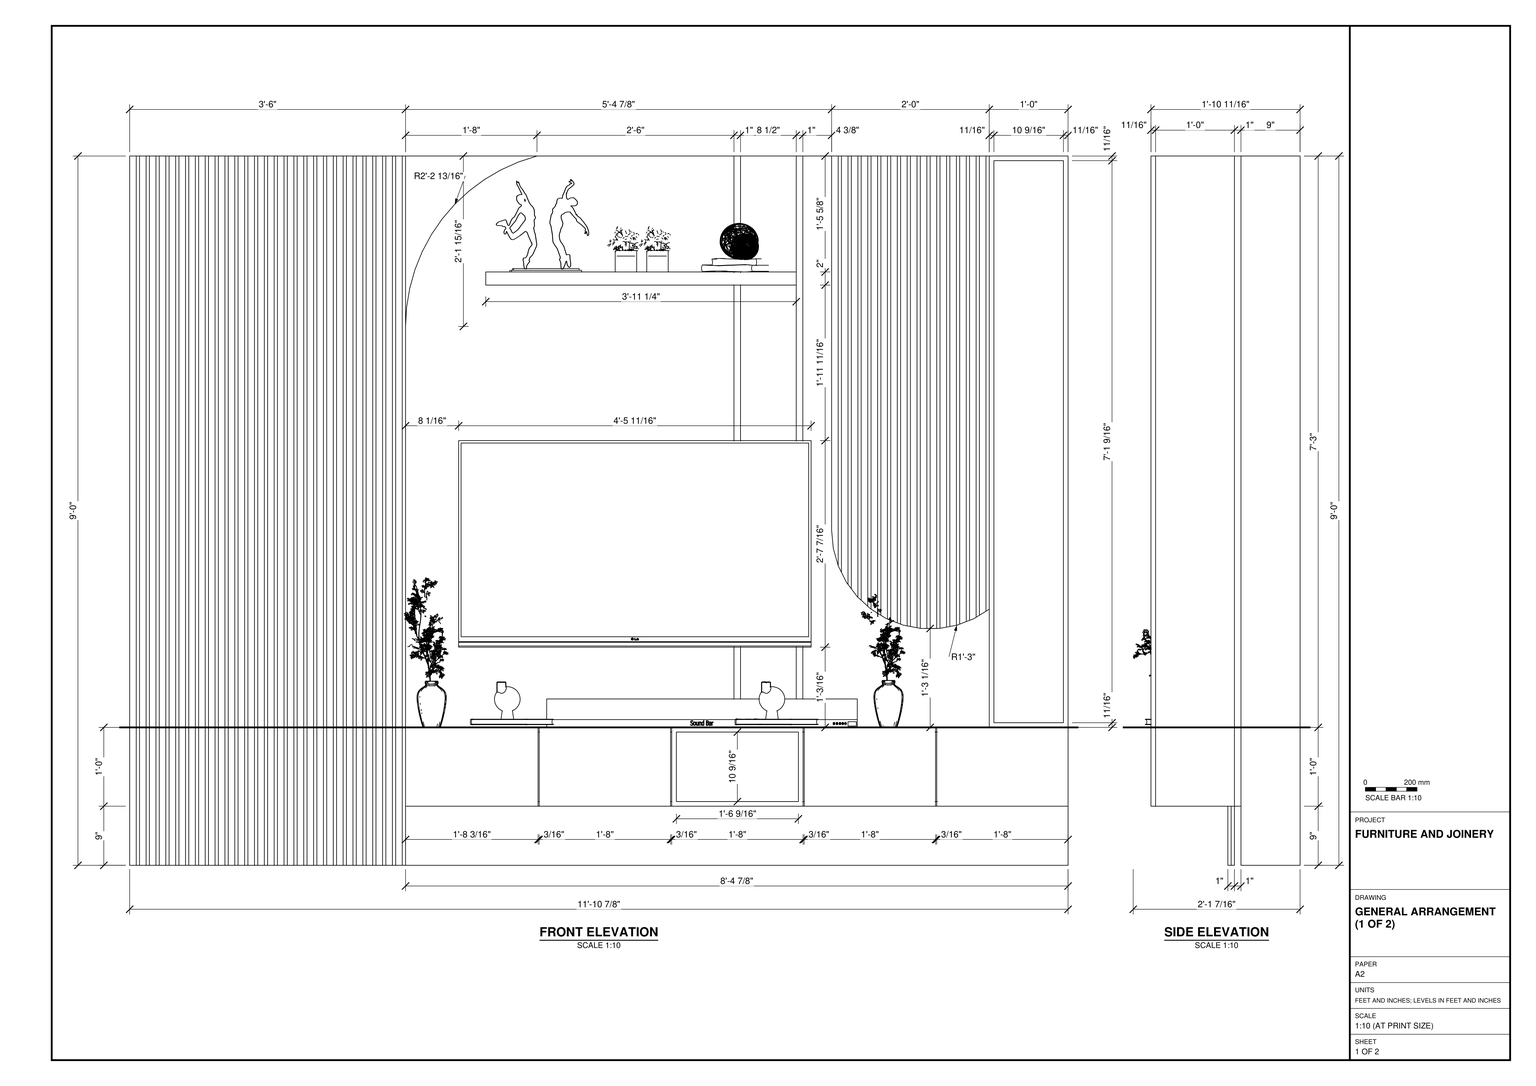
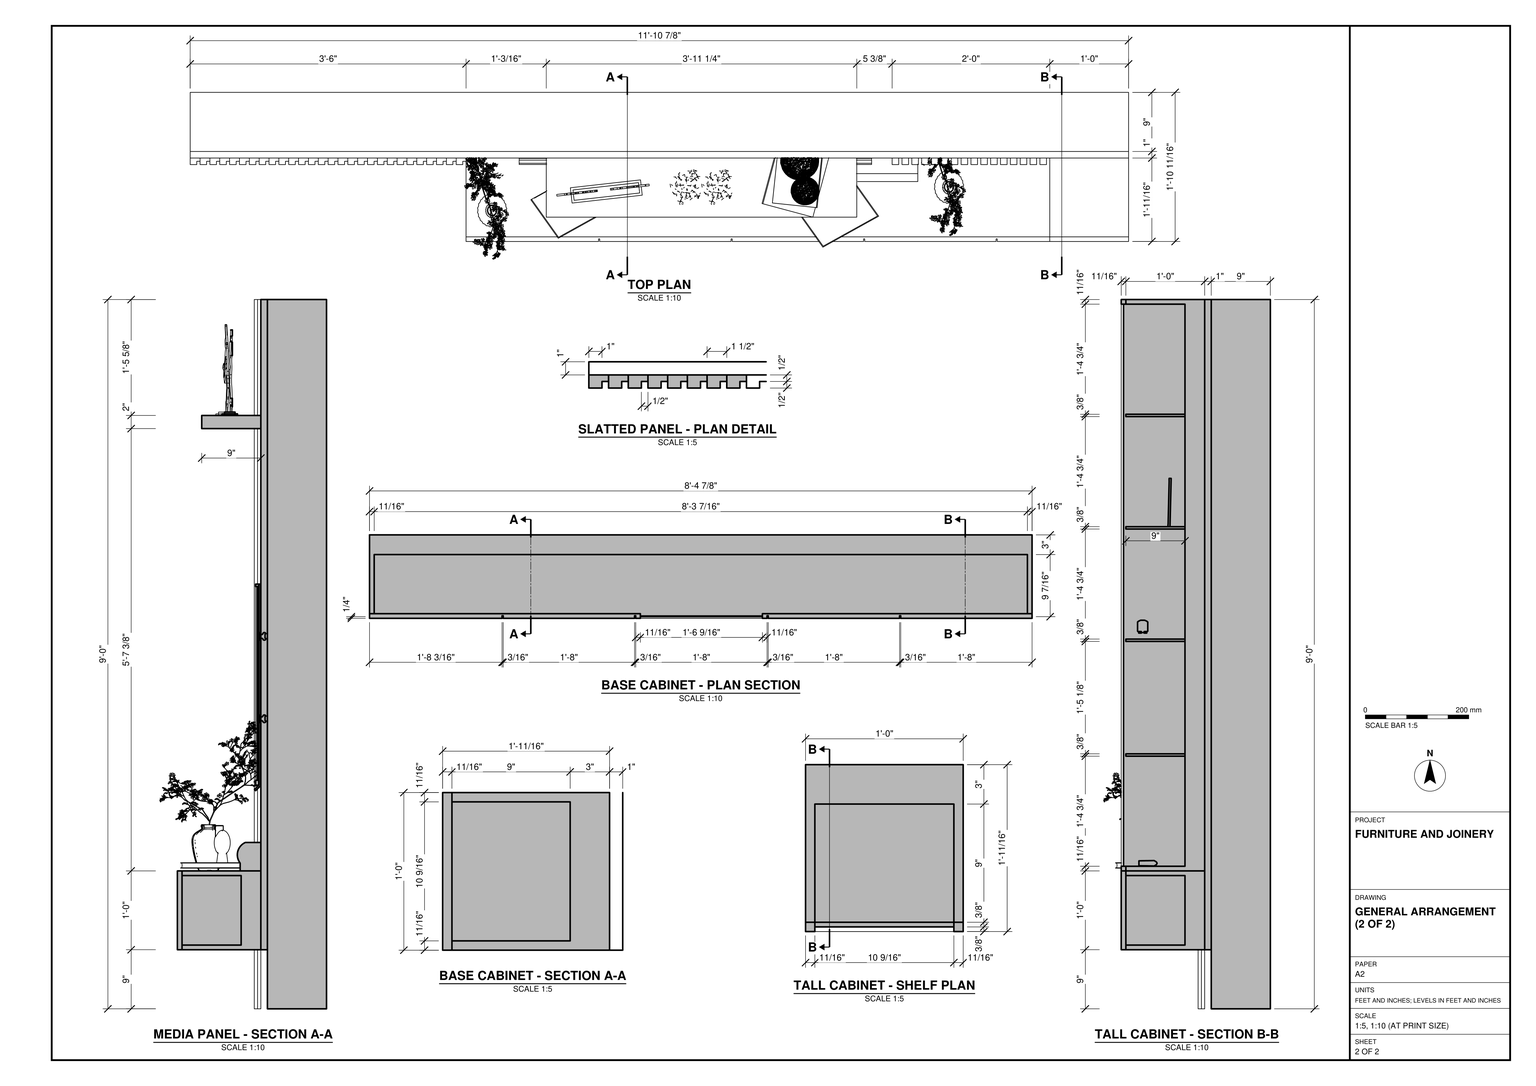
Build the media wall in SketchUp from task_files/diagram_01.pdf. Work in feet and inches, using the floor as the ±0'-0" datum. The complete assembly is 11'-10 7/8" wide, 2'-1 7/16" deep and 9'-0" high. Use the front elevation to set out the panels and cabinet faces, and the plan and sections to establish their depths.

Model the 9" thick backing wall and the full-height slatted panel at the left. Form the projecting slats and intervening grooves as shown in the plan detail. Reproduce the curved line at the upper left of the central media panel, its narrow vertical divisions and the curved lower edge of the slatted panel on the right. Fit the tall, narrow cabinet against the right end, with its framed front and internal shelves.

Run the suspended base cabinet from the left slatted panel to the right end. Include the gaps between its fronts and the inset centre bay. Position the television between the upper display shelf and the base cabinet, with the soundbar below the television. Decor and loose items on the shelf and cabinet may be any suitable library components. Keep the backing wall and each joinery or equipment piece in separate groups or components, and use components for repeated parts. Save one SketchUp model as output_files/media_wall_with_slatted_panels_and_fitted_cabinetry.skp.

# SketchUp Ruby script. Lengths in inches.
U = 1.inch
M = Sketchup.active_model
def pt(a) = Geom::Point3d.new(a.map { |v| v * U })
def face(e, loops, mat)
  f = e.add_face(loops[0].map { |a| pt(a) })
  loops[1..].each { |l| e.add_face(l.map { |a| pt(a) }).erase! }
  f.material = f.back_material = mat if mat
  f
end
# faces: each face lists its corners as indices into pts; further lists are holes
def faces(e, pts, list, mat = nil) = list.each { |f| face(e, (f[0].is_a?(Array) ? f : [f]).map { |l| l.map { |i| pts[i] } }, mat) }
# xy, xz, yz: faces in a plane at the given z, y or x. An outline is a flat list of corners, or four numbers for a rectangle; further outlines are holes
def ring(l) = l.size == 4 ? [[l[0], l[1]], [l[2], l[1]], [l[2], l[3]], [l[0], l[3]]] : l.each_slice(2).to_a
def flat(e, list, mat, &to3) = list.each { |f| face(e, (f[0].is_a?(Array) ? f : [f]).map { |l| ring(l).map { |u, v| to3.(u, v) } }, mat) }
def xy(e, z, list, mat = nil) = flat(e, list, mat) { |x, y| [x, y, z] }
def xz(e, y, list, mat = nil) = flat(e, list, mat) { |x, z| [x, y, z] }
def yz(e, x, list, mat = nil) = flat(e, list, mat) { |y, z| [x, y, z] }
def lines(e, pts, list) = list.each { |a, b| e.add_line(pt(pts[a]), pt(pts[b])) }
# prism: a flat outline (further loops are holes) pulled along v
def prism(e, loops, v, mat = nil)
  f = face(e, loops, mat); d = Geom::Vector3d.new(v.map { |x| x * U })
  f.pushpull(f.normal.samedirection?(d) ? d.length : -d.length)
end
def box(e, o, s, mat = nil) = prism(e, [[o, [o[0] + s[0], o[1], o[2]], [o[0] + s[0], o[1] + s[1], o[2]], [o[0], o[1] + s[1], o[2]]]], [0, 0, s[2]], mat)
def at(x, y, z, deg = 0) = Geom::Transformation.translation(pt([x, y, z])) * Geom::Transformation.rotation(ORIGIN, Z_AXIS, deg.degrees)
def axes(o, x, y, z) = Geom::Transformation.new([*x, 0, *y, 0, *z, 0, *pt(o).to_a, 1])
def part(name) = M.definitions.add(name)
# library, detail: a bought-in or finely detailed component or shape, given as its bounding box
def library(name, o, s) = part(name).tap { |d| box(d.entities, o, s) }
def detail(e, o, s) = box(e.add_group.entities, o, s)
def put(e, d, t, mat = nil) = e.add_instance(d, t).tap { |i| i.material = mat if mat }
def group(e, t, mat = nil) = e.add_group.tap { |g| g.transformation = t; g.material = mat if mat }.entities
root = M.entities
M.materials.add("C04_Amber_Sunshine").color = [255, 152, 49]
M.materials.add("Color_009").color = [0, 0, 0]
M.materials.add("Glass_Basic_01").color = [161, 173, 186]
M.materials["Glass_Basic_01"].alpha = 0.25
M.materials.add("M08_Obsidian_Black").color = [30, 30, 30]
M.materials.add("Plywood_01_1K").color = [125, 96, 64]
M.materials.add("[Color_000]2").color = [135, 140, 128]
c1 = library("Flat screen television",[0,8.92,0],[57.09,3.02,33.46])
c2 = library("Component114",[-82.06,-82.06,-129.5625],[164.12,164.12,259.1])
c3 = library("Component117",[-887.5,-1285.52,872.49],[3843.85,2719.29,5329.54])
c4 = library("Component119",[-554.81,-1390.41,779.52],[3610.96,2909.33,5473.88])
c5 = part("Component118")
put(c5.entities,c3,axes([-495.49,21.52,-677.71],[-0.13024,0.05973,0.15696],[-0.0368,-0.22453,0.01695],[0.17844,-0.01756,0.15474]))
put(c5.entities,c4,axes([-495.49,21.52,-677.71],[-0.13024,0.05973,0.15696],[-0.0368,-0.22453,0.01695],[0.17844,-0.01756,0.15474]))
c6 = part("Component116")
put(c6.entities,c2,axes([-124.16,15.74,-281.79],[-1.44088,0.62571,0],[-0.62571,-1.44088,0],[0,0,1.57088]))
put(c6.entities,c5,axes([19.67,96.68,265.57],[0.78615,0.27839,0],[0.27839,-0.78615,0],[0,0,0.83398]))
c7 = part("Component115")
put(c7.entities,c6,at(176.39,-15.27,-335.67))
c8 = library("Component124",[-34.71,-73.39,-113.66],[69.42,146.78,227.32])
c9 = library("Component126",[-109.42,-139.7,-27.27],[219.95,281.4,27.83])
c10 = library("Component128",[-218.98,-37.49,7.99],[213.01,261.68,22.71])
c11 = part("Component127")
put(c11.entities,c9,at(-0.56,-1,27.27))
put(c11.entities,c10,axes([112.41,-97.69,-5.43],[1,0,0],[0,1.0465,0],[0,0,1]))
c12 = part("Component125")
put(c12.entities,c8,axes([-16.9,-33.42,-7.27],[-0.38375,-0.70679,0],[-0.70679,0.38375,0],[0,0,0.80425]))
put(c12.entities,c11,axes([0,0,-117.43],[0.41792,0.87796,0],[0.87796,-0.41792,0],[0,0,0.97235]))
c13 = library("SoundBar",[0,0,0],[61.42,3.58,4.33])
c14 = library("dançarinos",[1.14,-1.57,0.12],[22.8,3.55,21.3])
c15 = library("Books and ornaments",[0,0,0],[11.85,7.68,6.68])
c16 = part("Group10\#1")
xy(c16.entities,0,[[-11,-26.41,-11.75,-23.78,-12,-21.03,-12,35.97,-11,35.97]])
xy(c16.entities,1,[[-11,-26.41,-11,35.97,-12,35.97,-12,-21.03,-11.75,-23.78]])
xz(c16.entities,35.97,[[-12,0,-11,1]])
yz(c16.entities,-12,[[-21.03,0,35.97,1]])
yz(c16.entities,-11,[[-26.41,0,35.97,1]])
c17 = part("Group11\#1")
xy(c17.entities,0,[[-9.5,-29.26,-9.76,-28.92,-10.5,-27.43,-10.5,35.97,-9.5,35.97]])
xy(c17.entities,1,[[-9.5,-29.26,-9.5,35.97,-10.5,35.97,-10.5,-27.43,-9.76,-28.92]])
xz(c17.entities,35.97,[[-10.5,0,-9.5,1]])
yz(c17.entities,-10.5,[[-27.43,0,35.97,1]])
yz(c17.entities,-9.5,[[-29.26,0,35.97,1]])
c18 = part("Group12\#1")
xy(c18.entities,0,[[-8,-31.21,-8.1,-31.125,-9,-29.92,-9,35.97,-8,35.97]])
xy(c18.entities,1,[[-8,-31.21,-8,35.97,-9,35.97,-9,-29.92,-8.1,-31.125]])
xz(c18.entities,35.97,[[-9,0,-8,1]])
yz(c18.entities,-9,[[-29.92,0,35.97,1]])
yz(c18.entities,-8,[[-31.21,0,35.97,1]])
c19 = part("Group13\#1")
prism(c19.entities,[[[-7.5,-31.67,0],[-7.5,35.97,0],[-6.5,35.97,0],[-6.5,-32.58,0]]],[0,0,1])
c20 = part("Group14\#1")
prism(c20.entities,[[[-6,-33.02,0],[-6,35.97,0],[-5,35.97,0],[-5,-33.64,0]]],[0,0,1])
c21 = part("Group15\#1")
xy(c21.entities,0,[[-3.5,-34.53,-3.71,-34.45,-4.5,-33.95,-4.5,35.97,-3.5,35.97]])
xy(c21.entities,1,[[-3.5,-34.53,-3.5,35.97,-4.5,35.97,-4.5,-33.95,-3.71,-34.45]])
xz(c21.entities,35.97,[[-4.5,0,-3.5,1]])
yz(c21.entities,-4.5,[[-33.95,0,35.97,1]])
yz(c21.entities,-3.5,[[-34.53,0,35.97,1]])
c22 = part("Group16\#1")
prism(c22.entities,[[[-3,-34.72,0],[-3,35.97,0],[-2,35.97,0],[-2,-35.11,0]]],[0,0,1])
c23 = part("Group17\#1")
xy(c23.entities,0,[[-0.5,-35.57,-1.13,-35.45,-1.5,-35.31,-1.5,35.97,-0.5,35.97]])
xy(c23.entities,1,[[-0.5,-35.57,-0.5,35.97,-1.5,35.97,-1.5,-35.31,-1.13,-35.45]])
yz(c23.entities,-1.5,[[-35.31,0,35.97,1]])
yz(c23.entities,-0.5,[[-35.57,0,35.97,1]])
c24 = part("Group18\#1")
prism(c24.entities,[[[1,35.97,0],[1,-35.85,0],[0,-35.66,0],[0,35.97,0]]],[0,0,1])
c25 = part("Group19\#1")
xy(c25.entities,0,[[2.5,-35.97,1.58,-35.96,1.5,-35.95,1.5,35.97,2.5,35.97]])
xy(c25.entities,1,[[2.5,-35.97,2.5,35.97,1.5,35.97,1.5,-35.95,1.58,-35.96]])
xz(c25.entities,35.97,[[1.5,0,2.5,1]])
yz(c25.entities,1.5,[[-35.95,0,35.97,1]])
yz(c25.entities,2.5,[[-35.97,0,35.97,1]])
c26 = part("Group20\#1")
box(c26.entities,[3,-35.97,0],[1,71.94,1])
c27 = part("Group21\#1")
prism(c27.entities,[[[4.5,-35.94,0],[4.5,35.97,0],[5.5,35.97,0],[5.5,-35.76,0]]],[0,0,1])
c28 = part("Group22\#1")
prism(c28.entities,[[[7,35.97,0],[7,-35.48,0],[6,-35.67,0],[6,35.97,0]]],[0,0,1])
c29 = part("Group23\#1")
prism(c29.entities,[[[8.5,35.97,0],[8.5,-34.92,0],[7.5,-35.3,0],[7.5,35.97,0]]],[0,0,1])
c30 = part("Group24\#1")
xy(c30.entities,0,[[9,-34.73,9,35.97,10,35.97,10,-34.26,9.65,-34.48]])
xy(c30.entities,1,[[9,-34.73,9.65,-34.48,10,-34.26,10,35.97,9,35.97]])
yz(c30.entities,9,[[-34.73,0,35.97,1]])
yz(c30.entities,10,[[-34.26,0,35.97,1]])
c31 = part("Group25\#1")
prism(c31.entities,[[[11.5,35.97,0],[11.5,-33.34,0],[10.5,-33.95,0],[10.5,35.97,0]]],[0,0,1])
c32 = part("Group26\#1")
yz(c32.entities,12,[[-33.03,0,35.97,1]])
c33 = part("Group8\#1")
put(c33.entities,c16,at(0,0,0))
put(c33.entities,c17,at(0,0,0))
put(c33.entities,c18,at(0,0,0))
put(c33.entities,c19,at(0,0,0))
put(c33.entities,c20,at(0,0,0))
put(c33.entities,c21,at(0,0,0))
put(c33.entities,c22,at(0,0,0))
put(c33.entities,c23,at(0,0,0))
put(c33.entities,c24,at(0,0,0))
put(c33.entities,c25,at(0,0,0))
put(c33.entities,c26,at(0,0,0))
put(c33.entities,c27,at(0,0,0))
put(c33.entities,c28,at(0,0,0))
put(c33.entities,c29,at(0,0,0))
put(c33.entities,c30,at(0,0,0))
put(c33.entities,c31,at(0,0,0))
put(c33.entities,c32,at(0,0,0))
c34 = part("Vertical wall slat")
xy(c34.entities,0,[[0,0,1,1],[1,0.5,1.5,1]])
xy(c34.entities,108,[[0,0,1,0,1,0.5,1.5,0.5,1.5,1,0,1]])
xz(c34.entities,0,[[0,0,1,108]])
xz(c34.entities,0.5,[[1,0,1.5,108]])
yz(c34.entities,0,[[0,0,1,108]])
yz(c34.entities,1,[[0,0,0.5,108]])
yz(c34.entities,1.5,[[0.5,0,1,108]])
c35 = part("Group\#9")
box(c35.entities,[0,0,0],[10.58,9,0.35])
c36 = library("Group7\#2",[0.82,-1.15,-0.02],[1.93,1.97,2.94])
c37 = library("Groupe\#10",[0,0,0],[43.68,4.59,18.71])
c38 = part("Agrupar\#3")
xy(c38.entities,21.7,[[0.99,0.93,21.68,0.97]])
yz(c38.entities,0,[[0.55,0,0,22.67,0.94,22.69,1.5,0.02]],"[Color_000]2")
yz(c38.entities,0.99,[[1.44,1.01,1.47,1.02,0.97,21.7,0.93,21.7]])
yz(c38.entities,21.68,[[1.44,1.01,0.93,21.7,0.97,21.7,1.47,1.02]])
yz(c38.entities,22.68,[[0.55,0,1.5,0.02,0.94,22.69,0,22.67]],"[Color_000]2")
p = [[0,0.55,0],[22.68,0.55,0],[22.68,0,22.67],[0,0,22.67],[0,1.5,0.02],[22.68,1.5,0.02],
  [0,0.94,22.69],[22.68,0.94,22.69],[21.68,1.47,1.02],[21.68,0.97,21.7],[0.99,0.97,21.7],[0.99,1.47,1.02],
  [21.68,0.93,21.7],[21.68,1.44,1.01],[0.99,1.44,1.01],[0.99,0.93,21.7]]
faces(c38.entities,p,[[0,1,2,3],[4,5,1,0],[7,6,3,2]],"[Color_000]2")
faces(c38.entities,p,[[[5,4,6,7],[8,9,10,11]],[12,13,14,15],[8,11,14,13]])
c39 = part("Agrupar\#30")
xy(c39.entities,14.62,[[0.51,0.6,16.18,0.64]])
yz(c39.entities,0,[[0.42,0,0,15.11,0.63,15.13,1.05,0.02]],"Color_009")
yz(c39.entities,0.51,[[1,0.52,1.04,0.53,0.64,14.62,0.6,14.62]])
yz(c39.entities,16.18,[[1,0.52,0.6,14.62,0.64,14.62,1.04,0.53]])
yz(c39.entities,16.69,[[0.42,0,1.05,0.02,0.63,15.13,0,15.11]],"Color_009")
p = [[0,0.42,0],[16.69,0.42,0],[16.69,0,15.11],[0,0,15.11],[16.69,1.05,0.02],[0,1.05,0.02],
  [0,0.63,15.13],[16.69,0.63,15.13],[16.18,0.64,14.62],[0.51,0.64,14.62],[0.51,1.04,0.53],[16.18,1.04,0.53],
  [0.51,0.6,14.62],[16.18,0.6,14.62],[16.18,1,0.52],[0.51,1,0.52]]
faces(c39.entities,p,[[0,1,2,3],[4,1,0,5],[2,7,6,3]],"Color_009")
faces(c39.entities,p,[[[4,5,6,7],[8,9,10,11]],[12,13,14,15],[11,10,15,14]])
c40 = library("Group\#263",[-0.77,-0.82,0],[7.28,10.35,17.46])
c41 = library("Group\#264",[0,0,0],[5.61,9.8,6.92])
put(root,c1,axes([103.75,22.95,33.21],[-0.94,0,0],[0,-0.94,0],[0,0,0.94]))
put(root,c7,axes([45.98,3.7,35.3],[0,0.01977,0],[-0.01747,0,0],[0,0,0.01747]))
put(root,c12,axes([58.2,5.79,25.2],[-0.01967,-0.02738,0],[0.03099,-0.01737,0],[0,0,0.03242]))
put(root,c7,axes([115.54,7.28,35.41],[0,0.01977,0],[-0.01747,0,0],[0,0,0.01747]))
put(root,c12,axes([98.49,4.43,25.2],[-0.01967,-0.02738,0],[0.03099,-0.01737,0],[0,0,0.03242]))
put(root,c13,axes([63.49,9.125,21],[0.77,0,0],[0,1,0],[0,0,1]))
put(root,c14,axes([70.6,8.5625,90.27],[-0.61653,-0.06916,0],[0.07357,-0.65589,0],[0,0,0.66]))
put(root,c15,axes([90.22,18.56,90.35],[-0.28729,-1.07218,0],[1.07218,-0.28729,0],[0,0,1.11]))
put(root,c15,axes([134.57,13.23,21.71],[-0.2327,-0.86846,0],[0.86846,-0.2327,0],[0,0,0.8991]))
g1 = group(root,at(0,13.71,0))
box(g1,[0,0,0],[142.87,9,108])
g2 = group(root,at(0,12.71,0))
xy(g2,9,[[0,0,142.87,1]])
xy(g2,108,[[0,0,142.87,1]])
xz(g2,0,[[0,9,42,108],[42,9,142.87,9,142.87,108,130.87,108,130.87,39,128.52,37.55,125.9375,36.5625,123.22,36.0625,120.45,36.07,117.74,36.58,115.16,37.58,112.82,39.04,110.78,40.91,109.11,43.11,107.88,45.59,107.125,48.25,106.87,51,106.87,108,102.49,108,102.49,21,101.49,21,101.49,108,93,108,93,21,92,21,92,108,62.01,108,59.22,107.1,56.54,105.9,54.01,104.41,51.65,102.66,49.5,100.66,47.59,98.4375,45.92,96.02,44.53,93.43,43.43,90.71,42.64,87.88,42.16,84.98,42,82.05],[123.22,36.0625,125.9375,36.5625,128.52,37.55,130.87,39,130.87,108,106.87,108,106.87,51,107.125,48.25,107.88,45.59,109.11,43.11,110.78,40.91,112.82,39.04,115.16,37.58,117.74,36.58,120.45,36.07],[42,82.05,42.16,84.98,42.64,87.88,43.43,90.71,44.53,93.43,45.92,96.02,47.59,98.4375,49.5,100.66,51.65,102.66,54.01,104.41,56.54,105.9,59.22,107.1,62.01,108,42,108]])
xz(g2,0,[[92,21,93,108],[101.49,21,102.49,108]],"C04_Amber_Sunshine")
xz(g2,1,[[0,9,142.87,108]])
yz(g2,0,[[0,9,1,108]])
yz(g2,142.87,[[0,9,1,108]])
put(g2,c33,axes([118.87,0,72.03],[1,0,0],[0,0,1],[0,-1,0]),"Plywood_01_1K")
g3 = group(root,at(0,11.71,0),"Plywood_01_1K")
put(g3,c34,at(1.5,0,0))
put(g3,c34,at(0,0,0))
put(g3,c34,at(3,0,0))
put(g3,c34,at(4.5,0,0))
put(g3,c34,at(6,0,0))
put(g3,c34,at(7.5,0,0))
put(g3,c34,at(9,0,0))
put(g3,c34,at(10.5,0,0))
put(g3,c34,at(12,0,0))
put(g3,c34,at(13.5,0,0))
put(g3,c34,at(15,0,0))
put(g3,c34,at(16.5,0,0))
put(g3,c34,at(18,0,0))
put(g3,c34,at(19.5,0,0))
put(g3,c34,at(21,0,0))
put(g3,c34,at(22.5,0,0))
put(g3,c34,at(24,0,0))
put(g3,c34,at(25.5,0,0))
put(g3,c34,at(27,0,0))
put(g3,c34,at(28.5,0,0))
put(g3,c34,at(30,0,0))
put(g3,c34,at(31.5,0,0))
put(g3,c34,at(33,0,0))
put(g3,c34,at(34.5,0,0))
put(g3,c34,at(36,0,0))
put(g3,c34,at(37.5,0,0))
put(g3,c34,at(39,0,0))
put(g3,c34,at(40.5,0,0))
g4 = group(root,at(42,0.71,9))
xy(g4,0,[[0,0,100.87,12]])
xy(g4,0.71,[[0.71,0,100.16,9]])
xy(g4,11.29,[[0.71,0,100.16,9]])
xy(g4,12,[[0,0,100.87,12]])
xz(g4,0,[[[0,0,100.87,12],[0.71,0.71,100.16,11.29]]])
xz(g4,9,[[0.71,0.71,100.16,11.29]])
xz(g4,12,[[0,0,100.87,12]])
yz(g4,0,[[0,0,12,12]])
yz(g4,0.71,[[0,0.71,9,11.29]])
yz(g4,100.16,[[0,0.71,9,11.29]])
yz(g4,100.87,[[0,0,12,12]])
g5 = group(root,at(54.21,0.71,88.35),"Plywood_01_1K")
box(g5,[0,3,0],[47.28,9,2])
g6 = group(root,at(42,0,9))
xy(g6,0,[[0,0,0,0.71,100.87,0.71,100.87,0,80.875,0,80.875,0.4,80.7,0.4,80.7,0,60.7,0,60.7,0.4,60.52,0.4,60.52,0,40.53,0,40.53,0.4,40.35,0.4,40.35,0,20.35,0,20.35,0.4,20.17,0.4,20.17,0]])
xy(g6,0.71,[[41.23,0,59.8125,0.71]],"M08_Obsidian_Black")
xy(g6,11.29,[[41.23,0,59.8125,0.71]],"M08_Obsidian_Black")
xy(g6,12,[[0,0,20.17,0,20.17,0.4,20.35,0.4,20.35,0,40.35,0,40.35,0.4,40.53,0.4,40.53,0,60.52,0,60.52,0.4,60.7,0.4,60.7,0,80.7,0,80.7,0.4,80.875,0.4,80.875,0,100.87,0,100.87,0.71,0,0.71]])
xz(g6,0,[[0,0,20.17,12],[20.35,0,40.35,12],[60.7,0,80.7,12],[80.875,0,100.87,12]])
xz(g6,0,[[[40.53,0,60.52,12],[41.23,0.71,59.8125,11.29]]],"M08_Obsidian_Black")
xz(g6,0.4,[[20.17,0,20.35,12],[40.35,0,40.53,12],[60.52,0,60.7,12],[80.7,0,80.875,12]])
xz(g6,0.71,[[[0,0,100.87,12],[41.23,0.71,59.8125,11.29]]])
yz(g6,0,[[0,0,0.71,12]])
yz(g6,20.17,[[0,0,0.4,12]])
yz(g6,20.35,[[0,0,0.4,12]])
yz(g6,40.35,[[0,0,0.4,12]])
yz(g6,40.53,[[0,0,0.4,12]])
yz(g6,41.23,[[0,0.71,0.71,11.29]],"M08_Obsidian_Black")
yz(g6,59.8125,[[0,0.71,0.71,11.29]],"M08_Obsidian_Black")
yz(g6,60.52,[[0,0,0.4,12]])
yz(g6,60.7,[[0,0,0.4,12]])
yz(g6,80.7,[[0,0,0.4,12]])
yz(g6,80.875,[[0,0,0.4,12]])
yz(g6,100.87,[[0,0,0.71,12]])
g7 = group(root,at(83.23,0.25,9.71),"Glass_Basic_01")
box(g7,[0,0,0],[18.58,0.1,10.58])
g8 = group(root,at(130.87,0.71,21))
g9 = group(g8,at(0,0,0))
xy(g9,0,[[0,0,12,12]])
xy(g9,0.71,[[0.71,0,11.29,9]])
xy(g9,86.29,[[0.71,0,11.29,9]])
xy(g9,87,[[0,0,12,12]])
xz(g9,0,[[[0,0,12,87],[0.71,0.71,11.29,86.29]]])
xz(g9,9,[[0.71,0.71,11.29,86.29]])
xz(g9,12,[[0,0,12,87]])
yz(g9,0,[[0,0,12,87]])
yz(g9,0.71,[[0,0.71,9,86.29]])
yz(g9,11.29,[[0,0.71,9,86.29]])
yz(g9,12,[[0,0,12,87]])
put(g8,c35,at(0.71,0,34.94))
put(g8,c35,at(0.71,0,17.47))
put(g8,c35,at(0.71,0,52.06))
put(g8,c35,at(0.71,0,69.17))
put(root,c36,axes([131.66,2.92,39.11],[3.10942,0,0],[0,3.10942,0],[0,0,3.10942]))
put(root,c37,axes([141.97,2.49,56.27],[-0.2257,0,0],[0,0.33855,0],[0,0,0.2257]))
g10 = group(root,at(131.79,6.85,73.41))
put(g10,c38,axes([0,0.75,0.01],[0.34037,0,0],[0,-0.32416,0],[0,0,0.32416]),"[Color_000]2")
put(g10,c39,axes([4.65,0.34,0],[0.34037,0,0],[0,-0.32416,0],[0,0,0.32416]),"[Color_000]2")
put(root,c40,axes([139.72,3.93,90.53],[0,0.76,0],[-0.76,0,0],[0,0,0.76]))
put(root,c41,at(72.77,11.07,90.35,-90))
g11 = group(root,at(130.87,0,21))
g12 = group(g11,at(0,0,0))
prism(g12,[[[0,0,0],[12,0,0],[12,0,87],[0,0,87]],[[11.29,0,0.71],[0.71,0,0.71],[0.71,0,86.29],[11.29,0,86.29]]],[0,0.71,0],"M08_Obsidian_Black")
g13 = group(g11,at(0.71,0.35,0.71),"Glass_Basic_01")
xz(g13,0,[[0,0,10.58,85.58]])
